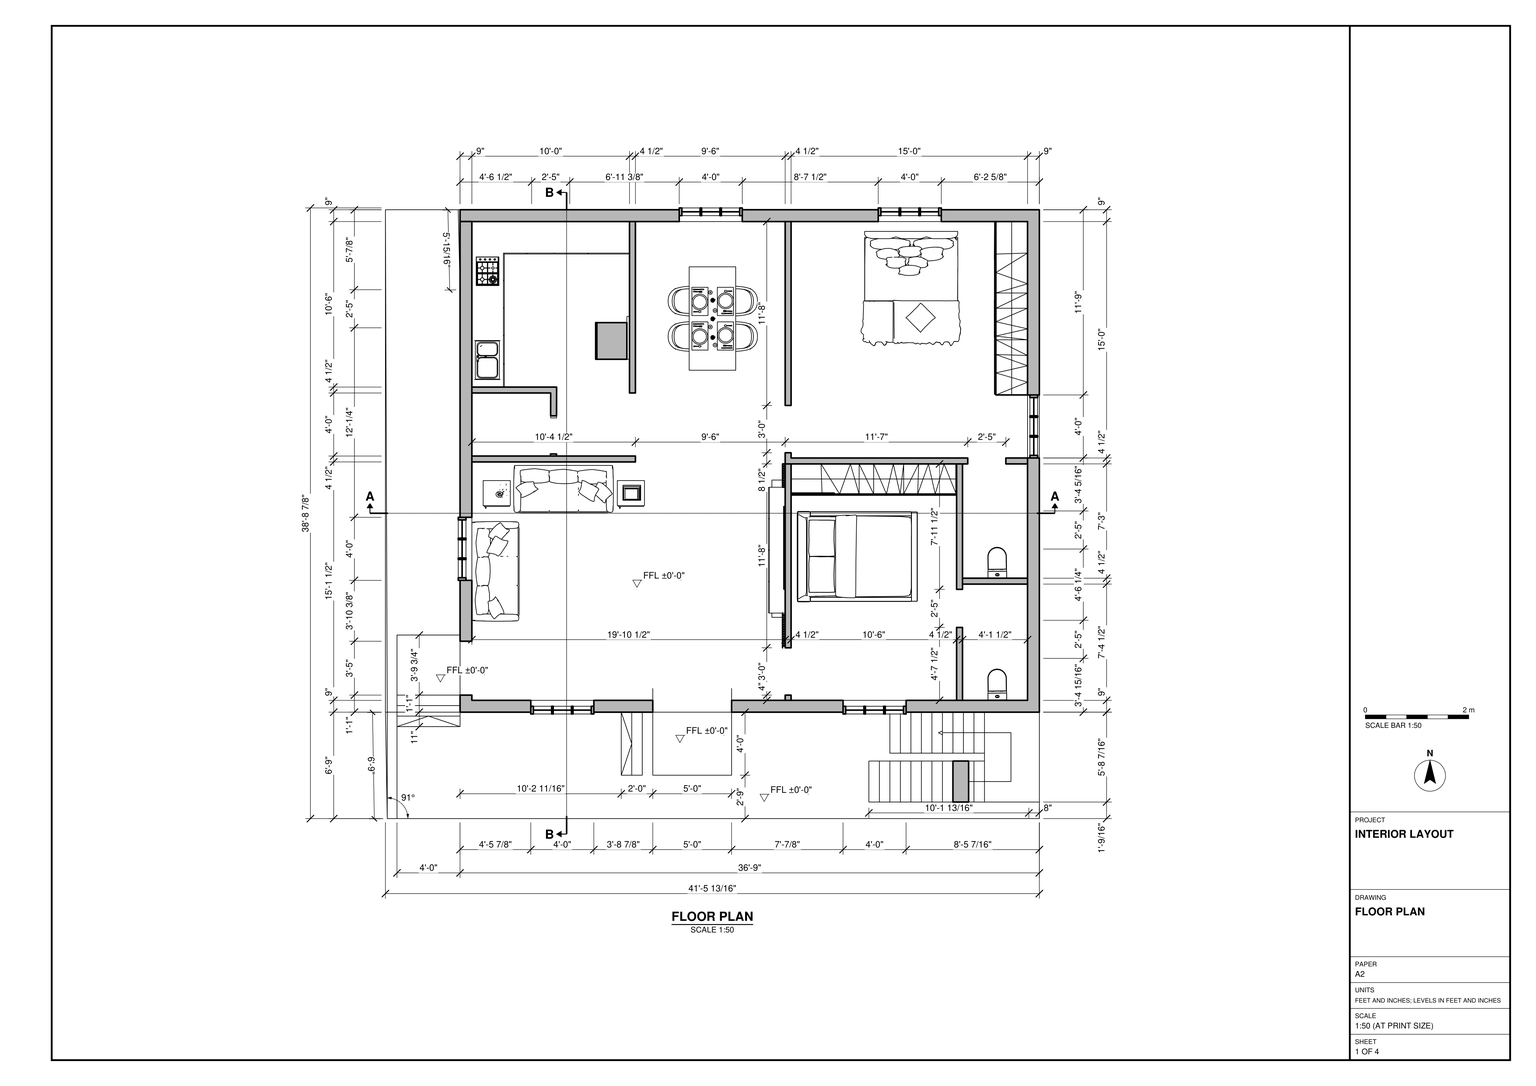
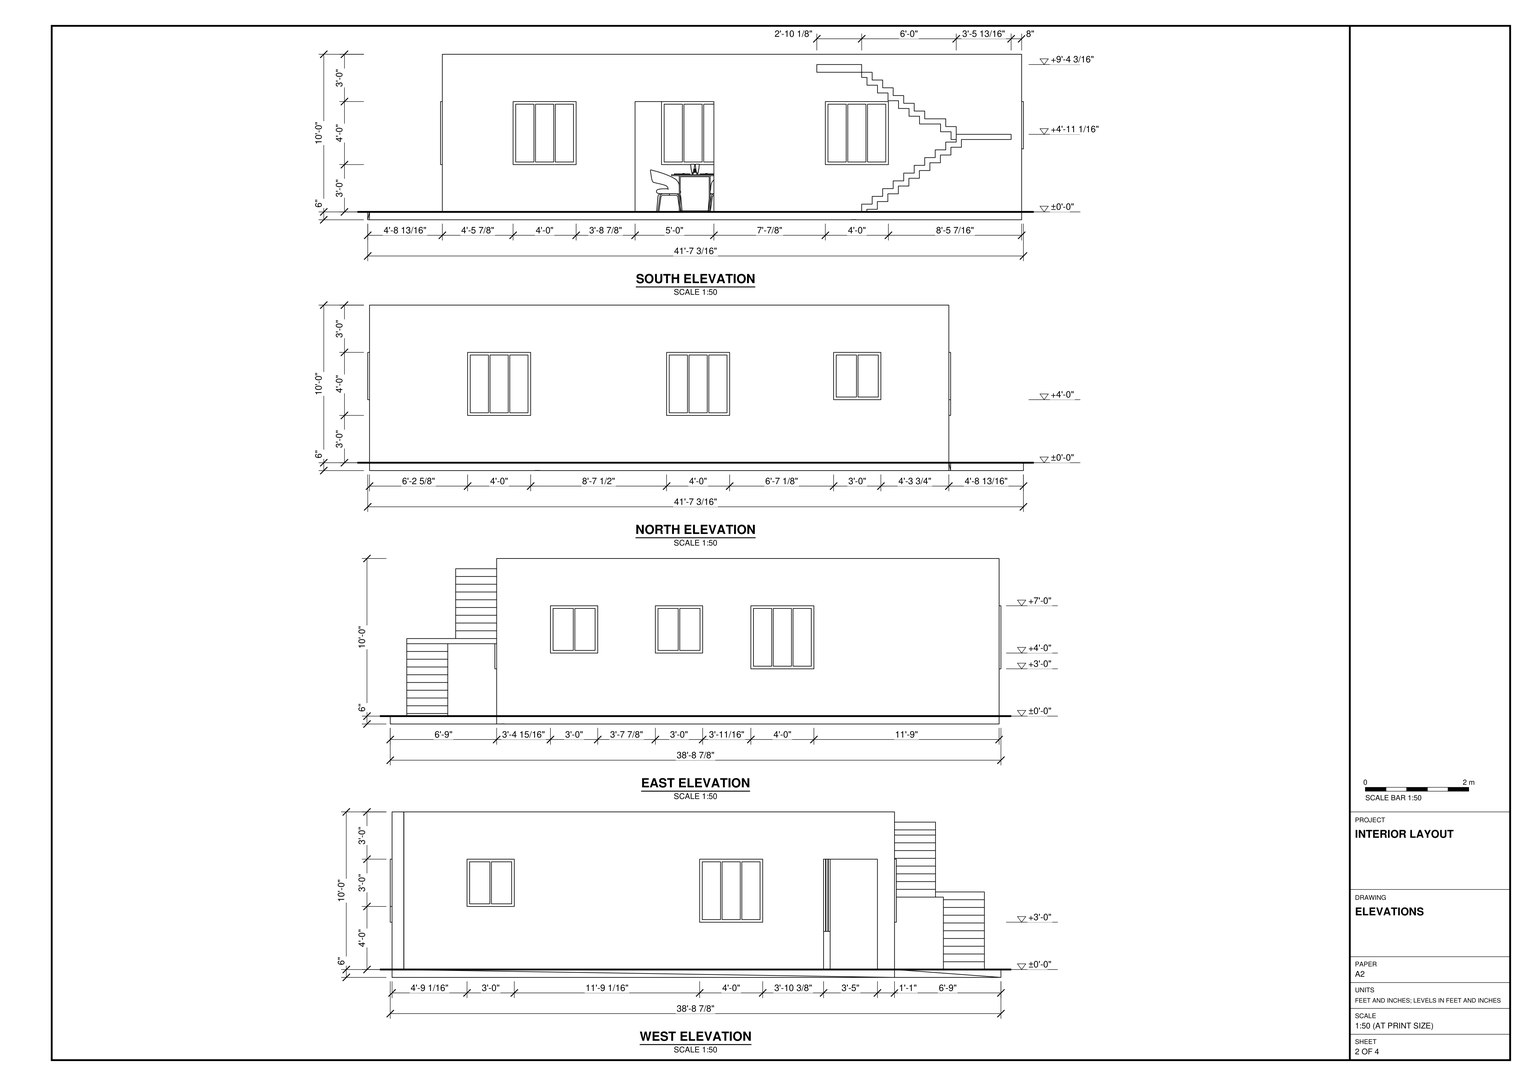
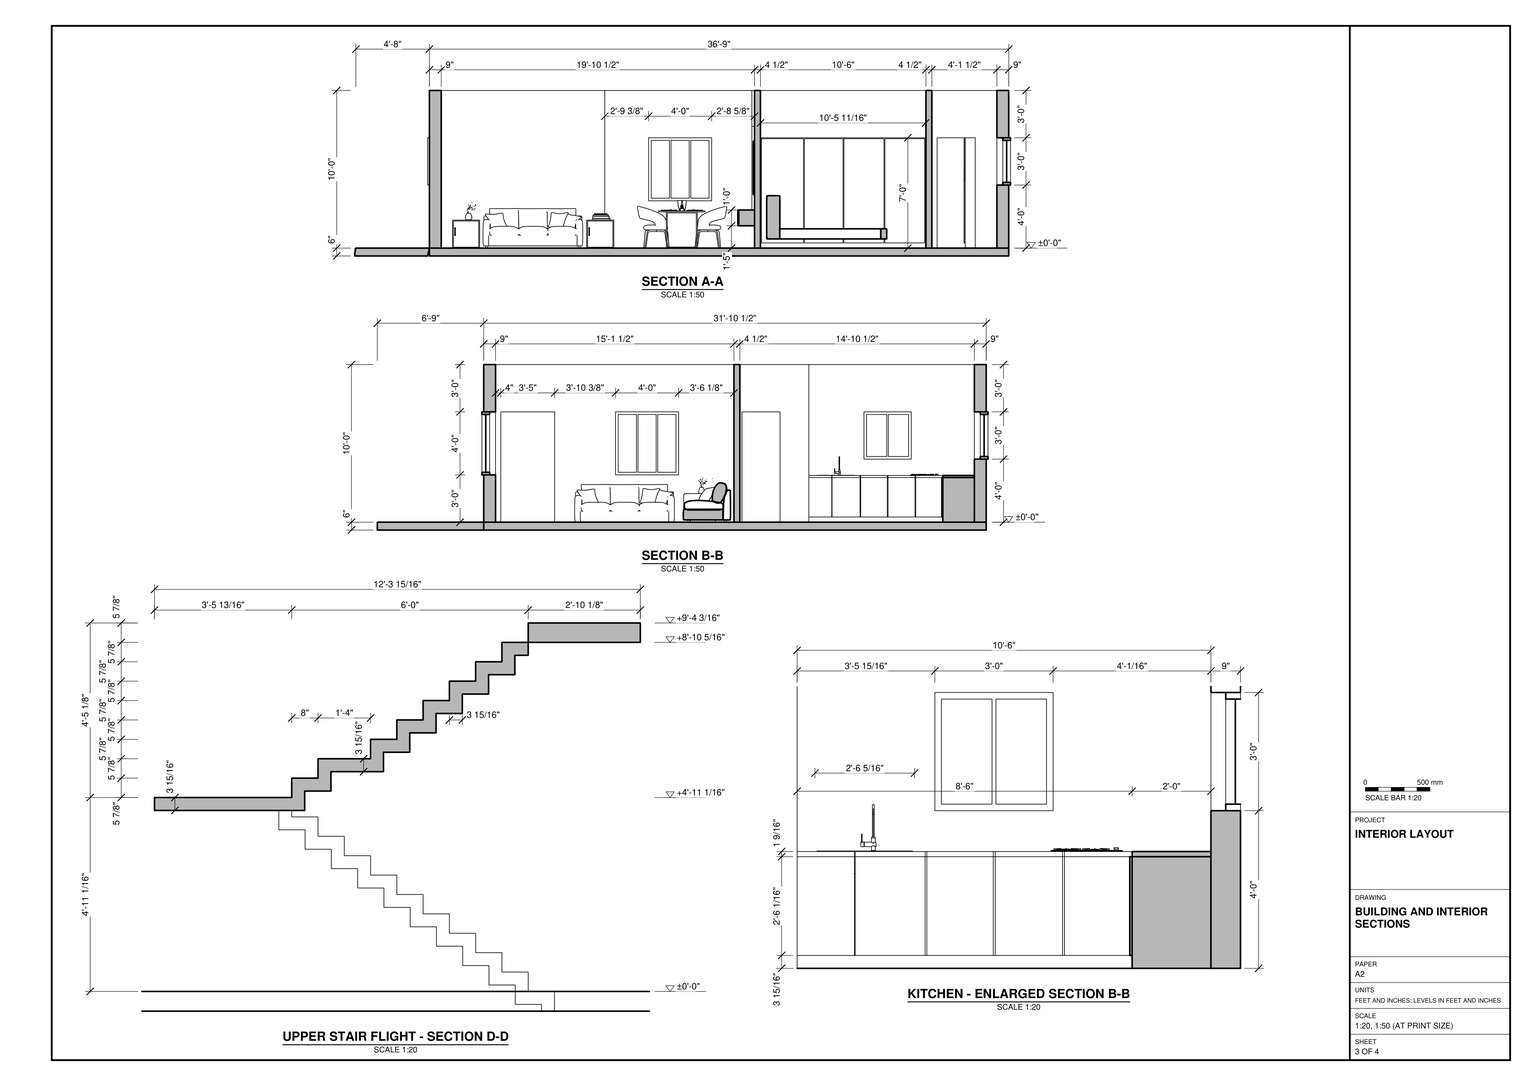
Build the single-storey residential layout in SketchUp from task_files/diagram_01.pdf. Work in feet and inches. Set the finished floor at ±0'-0". The overall model, including the projecting slab, is 41'-7 3/16" along x, 38'-8 7/8" along y and 10'-6" high.

Start with the 6" floor slab, including the portions extending beyond the south and west walls. Set out the 9" perimeter walls and the 4 1/2" partitions as drawn, with wall tops 10'-0" above the finished floor. Use the elevations to place the framed windows and exterior doorways. Build the exterior stair at the southeast corner with two flights that reverse direction at a shared landing.

Fit out the northwest kitchen with base cabinets, countertop, sink and cooktop. Place the dining table and chairs between the kitchen and the northeast bedroom, leaving the passage to the living area clear. Match the sofa arrangement in the southwest living area. Model both eastern bedrooms with their beds and fitted wardrobes, and include the two toilet compartments along the east wall.

Keep shell elements, the stair and each furniture or joinery piece in separate groups or components; use components for repeated parts. Decor and loose items, including lamps and appliances, may be any suitable library components. Save one SketchUp model as output_files/furnished_two_bedroom_layout_with_exterior_return_stair.skp.

# SketchUp Ruby script. Lengths in inches.
U = 1.inch
M = Sketchup.active_model
def pt(a) = Geom::Point3d.new(a.map { |v| v * U })
def face(e, loops, mat)
  f = e.add_face(loops[0].map { |a| pt(a) })
  loops[1..].each { |l| e.add_face(l.map { |a| pt(a) }).erase! }
  f.material = f.back_material = mat if mat
  f
end
# faces: each face lists its corners as indices into pts; further lists are holes
def faces(e, pts, list, mat = nil) = list.each { |f| face(e, (f[0].is_a?(Array) ? f : [f]).map { |l| l.map { |i| pts[i] } }, mat) }
# xy, xz, yz: faces in a plane at the given z, y or x. An outline is a flat list of corners, or four numbers for a rectangle; further outlines are holes
def ring(l) = l.size == 4 ? [[l[0], l[1]], [l[2], l[1]], [l[2], l[3]], [l[0], l[3]]] : l.each_slice(2).to_a
def flat(e, list, mat, &to3) = list.each { |f| face(e, (f[0].is_a?(Array) ? f : [f]).map { |l| ring(l).map { |u, v| to3.(u, v) } }, mat) }
def xy(e, z, list, mat = nil) = flat(e, list, mat) { |x, y| [x, y, z] }
def xz(e, y, list, mat = nil) = flat(e, list, mat) { |x, z| [x, y, z] }
def yz(e, x, list, mat = nil) = flat(e, list, mat) { |y, z| [x, y, z] }
def lines(e, pts, list) = list.each { |a, b| e.add_line(pt(pts[a]), pt(pts[b])) }
# prism: a flat outline (further loops are holes) pulled along v
def prism(e, loops, v, mat = nil)
  f = face(e, loops, mat); d = Geom::Vector3d.new(v.map { |x| x * U })
  f.pushpull(f.normal.samedirection?(d) ? d.length : -d.length)
end
def box(e, o, s, mat = nil) = prism(e, [[o, [o[0] + s[0], o[1], o[2]], [o[0] + s[0], o[1] + s[1], o[2]], [o[0], o[1] + s[1], o[2]]]], [0, 0, s[2]], mat)
def at(x, y, z, deg = 0) = Geom::Transformation.translation(pt([x, y, z])) * Geom::Transformation.rotation(ORIGIN, Z_AXIS, deg.degrees)
def axes(o, x, y, z) = Geom::Transformation.new([*x, 0, *y, 0, *z, 0, *pt(o).to_a, 1])
def part(name) = M.definitions.add(name)
# library, detail: a bought-in or finely detailed component or shape, given as its bounding box
def library(name, o, s) = part(name).tap { |d| box(d.entities, o, s) }
def detail(e, o, s) = box(e.add_group.entities, o, s)
def put(e, d, t, mat = nil) = e.add_instance(d, t).tap { |i| i.material = mat if mat }
def group(e, t, mat = nil) = e.add_group.tap { |g| g.transformation = t; g.material = mat if mat }.entities
root = M.entities
M.materials.add("2121 AP  X165 Dhaani-I").color = [217, 210, 92]
M.materials.add("2130 AP  X175 Sawan-I").color = [3, 168, 115]
M.materials.add("2186 AP  X202 Auspicious red-I").color = [192, 71, 86]
M.materials.add("Translucent_Glass_Gray1").color = [255, 255, 255]
M.materials["Translucent_Glass_Gray1"].alpha = 0.2
M.materials.add("Vicostone-BQ8740-Nero-Marquina-or-NERO-MARQUINAtm-CAN-or-US-").color = [21, 21, 22]
M.materials.add("[Chris_Shoe]").color = [23, 22, 22]
M.materials.add("[Color M05]").color = [114, 114, 114]
M.materials.add("[Color M08]").color = [30, 30, 30]
M.materials.add("[Color M09]").color = [0, 0, 0]
M.materials.add("[Tile Large Brown]").color = [193, 176, 158]
M.materials.add("[Translucent Glass Blue]").color = [100, 149, 237]
M.materials["[Translucent Glass Blue]"].alpha = 0.5
M.materials.add("[Wood Veneer 01]").color = [119, 69, 36]
c1 = part("new blockwindow")
p = [[-24,-4.5,0],[-24,4.5,0],[24,4.5,0],[24,-4.5,0],[24,-2,0],[-24,-2,0],
  [24,2,0],[-24,2,0]]
lines(c1.entities,p,[[0,1],[1,2],[2,3],[3,0],[4,5],[6,7]])
c2 = part("Bed - Queen")
p = [[22,23.6,0],[16.8,23.6,0],[22,38.8,0],[1.2,38.8,0],[1.2,25.6,0],[-1.2,38.8,0],
  [-1.2,25.6,0],[-22,38.8,0],[-22,25.6,0],[30,-40,0],[-30,-40,0],[-30,40,0],
  [14.8,23.2,0],[-30,23.2,0],[-30,25.6,0],[14.8,25.6,0],[30,40,0],[30,10.4,0],
  [14.8,10.4,0]]
lines(c2.entities,p,[[0,1],[2,0],[3,2],[4,3],[5,6],[7,5],[8,7],[9,10],[10,11],[12,13],[14,15],[11,16],
  [16,9],[17,15],[18,17],[15,18]])
c3 = library("Dining Set - 36 x 72 in.",[-45.5,-27.5,0],[91,55,0.01])
c4 = part("Sofa - Roundback 7 ft.")
p = [[12,-15.44,0],[12,10.4,0],[42,9,0],[42,-17,0],[36,-17,0],[36,5.53,0],
  [-12,-15.44,0],[-12,10.4,0],[-36,-17,0],[-42,-17,0],[-42,9,0],[-36,5.53,0],
  [-36,-15.44,0],[36,-15.44,0],[-36,3.62,0],[36,3.62,0],[28.96,7.49,0],[21.8125,9.02,0],
  [14.59,10.12,0],[7.31,10.78,0],[0,11,0],[-7.31,10.78,0],[-14.59,10.12,0],[-21.8125,9.02,0],
  [-28.96,7.49,0],[35.26,11.42,0],[28.37,13.42,0],[21.38,14.98,0],[14.3,16.1,0],[7.16,16.78,0],
  [0,17,0],[-7.16,16.78,0],[-14.3,16.1,0],[-21.38,14.98,0],[-28.37,13.42,0],[-35.26,11.42,0]]
lines(c4.entities,p,[[0,1],[2,3],[3,4],[4,5],[6,7],[8,9],[9,10],[8,11],[12,13],[14,15],[5,16],[16,17],
  [17,18],[18,19],[19,20],[20,21],[21,22],[22,23],[23,24],[24,11],[2,25],[25,26],[26,27],[27,28],
  [28,29],[29,30],[30,31],[31,32],[32,33],[33,34],[34,35],[35,10]])
c5 = library("Sink-double - 36 in top",[-18,-10.5,0],[36,21,0.01])
c6 = library("Range-Oven - 30 in top",[-15,-13,0],[30,26,0.01])
c7 = library("Dishwasher",[-12,-17.25,0],[24,34.5,0.01])
c8 = library("lamp",[-10.34,-9.52,0],[20.68,19.04,0.01])
c9 = library("Sofa 005",[-44.88,-17.99,0],[89.76,35.98,35.98])
c10 = library("1-POIGNEE CLC2",[-3.03,-0.375,0],[6.06,0.75,1.42])
c11 = library("2-VASEFLEURS CLC2",[-2.64,-4.18,0],[11.14,15.39,15.4375])
c12 = library("Stack of books",[0,0,0],[13.58,11.5,4.89])
c13 = part("Component\#1")
box(c13.entities,[0,0,0],[35.43,78.74,0.79],"Translucent_Glass_Gray1")
c14 = part("Rectangular frame")
prism(c14.entities,[[[29.53,5.91,0],[29.53,5.91,27.56],[5.91,5.91,27.56],[5.91,5.91,0]],[[28.74,5.91,0.79],[6.69,5.91,0.79],[6.69,5.91,26.77],[28.74,5.91,26.77]]],[0,3.9375,0],"[Color M08]")
c15 = library("chair 62",[0,0,0],[22.98,24.17,32.16])
c16 = library("Potted succulent",[-0.04,0,0],[3.63,3.68,4.41])
c17 = library("glass",[-1.4375,-1.4375,0],[2.875,2.875,7.95])
c18 = library("Bed 003",[-38.05,-87.1,0],[75.86,87.1,46.85])
c19 = library("Crowd Pleaser Bed",[-34.48,-45.67,0],[68.96,91.51,40.05])
c20 = library("Toilet",[-7.17,-23.62,0],[14.34,23.62,32.58])
c21 = part("Component")
g1 = group(c21.entities,at(263.61,28.98,0))
xy(g1,1.32,[[-23.76,-27.93,-22.86,0]])
xy(g1,30.41,[[-23.76,-24.34,-22.94,-3.73]])
xy(g1,32.16,[[-23.76,-27.93,-22.94,-24.34],[-23.76,-3.73,-22.94,0]])
xy(g1,32.68,[[-23.76,-27.93,-22.94,0]])
xy(g1,72.97,[[-23.76,-27.93,-22.86,0]])
xz(g1,-27.93,[[-23.76,1.32,-22.86,1.32,-22.86,72.97,-23.76,72.97,-23.76,32.68,-22.94,32.68,-22.94,32.16,-23.76,32.16]])
xz(g1,-24.34,[[-23.76,30.41,-22.94,32.16]])
xz(g1,-3.73,[[-23.76,30.41,-22.94,32.16]])
xz(g1,0,[[-23.76,1.32,-23.76,32.16,-22.94,32.16,-22.94,32.68,-23.76,32.68,-23.76,72.97,-22.86,72.97,-22.86,1.32]])
yz(g1,-23.76,[[-27.93,1.32,-27.93,32.16,-24.34,32.16,-24.34,30.41,-3.73,30.41,-3.73,32.16,0,32.16,0,1.32],[-27.93,32.68,0,72.97]])
yz(g1,-22.94,[[-24.34,30.41,-3.73,32.16],[-27.93,32.16,0,32.68]])
yz(g1,-22.86,[[-27.93,1.32,0,72.97]])
g2 = group(g1,at(-22.86,-1.74,75.13))
xy(g2,-75.13,[[0,-26.1875,22.86,1.72]])
xy(g2,-2.16,[[0,-26.1875,22.86,1.72]])
xz(g2,-26.1875,[[0,-75.13,22.86,-2.16]])
xz(g2,1.72,[[0,-75.13,22.86,-2.16]])
yz(g2,0,[[-26.1875,-75.13,1.72,-73.81],[1.72,-75.13,1.74,-73.81],[-26.1875,-73.81,1.72,-2.16]])
yz(g2,22.86,[[-26.1875,-75.13,1.72,-2.16]])
c22 = library("4-TABLE DE CUISSON CLC2",[-10.93,-8.66,0.2],[21.86,17.32,1.1])
c23 = library("2-EVIER M80 CLC2\#1",[-15.14,-9.87,-6.7],[30.32,19.69,21.06])
c24 = part("Group18\#1")
xy(c24.entities,0,[[121.34,276.07,116.84,276.08,116.84,277.59,121.34,277.58],[121.43,306.58,116.93,306.59,116.99,324,57,324,57,328.5,121.5,328.5]])
xy(c24.entities,84,[[121.34,277.58,116.84,277.59,116.93,306.59,121.43,306.58]])
xy(c24.entities,120,[[121.34,276.07,121.5,328.5,57,328.5,57,324,116.99,324,116.84,276.08]])
xz(c24.entities,324,[[57,0,116.99,120]])
xz(c24.entities,328.5,[[57,0,121.5,120]])
yz(c24.entities,57,[[324,0,328.5,120]])
# 1 loose lines left out
p = [[116.99,324,0],[116.93,306.59,0],[116.93,306.59,84],[116.84,277.59,84],[116.84,277.59,0],[116.84,276.08,0],
  [116.84,276.08,120],[116.99,324,120],[121.34,276.07,0],[121.34,276.07,120],[121.34,277.58,0],[121.34,277.58,84],
  [121.43,306.58,84],[121.43,306.58,0],[121.5,328.5,0],[121.5,328.5,120]]
faces(c24.entities,p,[[0,1,2,3,4,5,6,7],[8,9,6,5],[8,10,11,12,13,14,15,9],[4,3,11,10],[2,1,13,12]])
c25 = part("Group19\#1")
box(c25.entities,[57,271.5,0],[124.5,4.5,120])
c26 = part("Group21\#1")
box(c26.entities,[177,324,0],[4.5,130.5,120])
c27 = part("Group22\#1")
xy(c27.entities,0,[[295.5,270,295.5,278.5,300,278.5,300,274.5,434.5,274.5,434.5,270],[463.5,270,480,274.5],[295.5,314.5,300,454.5]])
xy(c27.entities,84,[[434.5,270,463.5,274.5],[295.5,278.5,300,314.5]])
xy(c27.entities,120,[[295.5,270,480,270,480,274.5,300,274.5,300,454.5,295.5,454.5]])
xz(c27.entities,270,[[295.5,0,434.5,0,434.5,84,463.5,84,463.5,0,480,0,480,120,295.5,120]])
xz(c27.entities,274.5,[[300,0,300,120,480,120,480,0,463.5,0,463.5,84,434.5,84,434.5,0]])
xz(c27.entities,278.5,[[295.5,0,300,84]])
xz(c27.entities,314.5,[[295.5,0,300,84]])
xz(c27.entities,454.5,[[295.5,0,300,120]])
yz(c27.entities,295.5,[[270,0,270,120,454.5,120,454.5,0,314.5,0,314.5,84,278.5,84,278.5,0]])
yz(c27.entities,300,[[274.5,0,278.5,0,278.5,84,314.5,84,314.5,0,454.5,0,454.5,120,274.5,120]])
yz(c27.entities,434.5,[[270,0,274.5,84]])
yz(c27.entities,463.5,[[270,0,274.5,84]])
yz(c27.entities,480,[[270,0,274.5,120]])
c28 = part("Group24\#1")
prism(c28.entities,[[[430.5,90,0],[430.5,145.5,0],[430.5,145.5,84],[430.5,174.5,84],[430.5,174.5,0],[430.5,270,0],[430.5,270,120],[430.5,90,120]]],[-4.5,0,0])
c29 = part("Group26\#1")
box(c29.entities,[430.5,178.5,0],[49.5,4.5,120])
c30 = library("Group\#2",[0,0,0],[100.17,68.42,0.01])
c31 = library("Group\#3",[0,0,0],[121.79,68.42,0.01])
c32 = library("Group\#6",[0,0,0],[121.79,68.42,118.11])
c33 = part("Group55\#3")
xy(c33.entities,0,[[-22,-22,-8.125,22],[-6.9375,-22,6.9375,22],[8.125,-22,22,22]])
c34 = part("Group54\#1")
prism(c34.entities,[[[-24,24,0],[24,24,0],[24,-24,0],[-24,-24,0]],[[-22,22,0],[-22,-22,0],[-8.125,-22,0],[-8.125,22,0]],[[6.9375,22,0],[-6.9375,22,0],[-6.9375,-22,0],[6.9375,-22,0]],[[22,-22,0],[22,22,0],[8.125,22,0],[8.125,-22,0]]],[0,0,5.875],"[Chris_Shoe]")
put(c34.entities,c33,at(0,0,2.9375))
c35 = part("Group57\#2")
xy(c35.entities,0,[[-22,-22,-8.125,22],[-6.9375,-22,6.9375,22],[8.125,-22,22,22]])
c36 = part("Group56\#1")
prism(c36.entities,[[[24,-24,0],[-24,-24,0],[-24,24,0],[24,24,0]],[[-22,22,0],[-22,-22,0],[-8.125,-22,0],[-8.125,22,0]],[[8.125,-22,0],[22,-22,0],[22,22,0],[8.125,22,0]],[[-6.9375,-22,0],[6.9375,-22,0],[6.9375,22,0],[-6.9375,22,0]]],[0,0,5.875],"[Chris_Shoe]")
put(c36.entities,c35,at(0,0,2.9375))
c37 = part("Group54\#2")
prism(c37.entities,[[[-24,24,0],[24,24,0],[24,-24,0],[-24,-24,0]],[[-22,22,0],[-22,-22,0],[-8.125,-22,0],[-8.125,22,0]],[[6.9375,22,0],[-6.9375,22,0],[-6.9375,-22,0],[6.9375,-22,0]],[[22,-22,0],[22,22,0],[8.125,22,0],[8.125,-22,0]]],[0,0,5.875],"[Chris_Shoe]")
put(c37.entities,c33,at(0,0,2.9375))
c38 = part("Group63\#2")
xy(c38.entities,0,[[-22,-22,-8.125,22],[-6.9375,-22,6.9375,22],[8.125,-22,22,22]])
c39 = part("Group62\#2")
prism(c39.entities,[[[-24,-24,0],[-24,24,0],[24,24,0],[24,-24,0]],[[6.9375,22,0],[-6.9375,22,0],[-6.9375,-22,0],[6.9375,-22,0]],[[8.125,22,0],[8.125,-22,0],[22,-22,0],[22,22,0]],[[-8.125,-22,0],[-8.125,22,0],[-22,22,0],[-22,-22,0]]],[0,0,5.875],"[Chris_Shoe]")
put(c39.entities,c38,at(0,0,2.9375))
c40 = part("Group65\#3")
xy(c40.entities,0,[[-22,-22,-8.125,22],[-6.9375,-22,6.9375,22],[8.125,-22,22,22]])
c41 = part("Group64\#1")
prism(c41.entities,[[[-24,-24,0],[-24,24,0],[24,24,0],[24,-24,0]],[[-6.9375,-22,0],[6.9375,-22,0],[6.9375,22,0],[-6.9375,22,0]],[[8.125,-22,0],[22,-22,0],[22,22,0],[8.125,22,0]],[[-22,-22,0],[-8.125,-22,0],[-8.125,22,0],[-22,22,0]]],[0,0,5.875],"[Chris_Shoe]")
put(c41.entities,c40,at(0,0,2.9375))
c42 = part("Group67\#2")
xy(c42.entities,0,[[-16,-16,-0.59,16],[0.59,-16,16,16]])
c43 = part("Group66\#1")
prism(c43.entities,[[[-18,18,0],[18,18,0],[18,-18,0],[-18,-18,0]],[[16,-16,0],[16,16,0],[0.59,16,0],[0.59,-16,0]],[[-0.59,16,0],[-16,16,0],[-16,-16,0],[-0.59,-16,0]]],[0,0,5.875],"[Chris_Shoe]")
put(c43.entities,c42,at(0,0,2.9375))
c44 = part("Group69\#3")
xy(c44.entities,0,[[-16,-16,-0.59,16],[0.59,-16,16,16]])
c45 = part("Group68\#1")
prism(c45.entities,[[[-18,18,0],[18,18,0],[18,-18,0],[-18,-18,0]],[[-16,-16,0],[-0.59,-16,0],[-0.59,16,0],[-16,16,0]],[[16,-16,0],[16,16,0],[0.59,16,0],[0.59,-16,0]]],[0,0,5.875],"[Chris_Shoe]")
put(c45.entities,c44,at(0,0,2.9375))
c46 = part("Group67\#3")
xy(c46.entities,0,[[-16,-16,-0.59,16],[0.59,-16,16,16]])
c47 = part("Group66\#2")
prism(c47.entities,[[[-18,18,0],[18,18,0],[18,-18,0],[-18,-18,0]],[[-16,-16,0],[-0.59,-16,0],[-0.59,16,0],[-16,16,0]],[[16,16,0],[0.59,16,0],[0.59,-16,0],[16,-16,0]]],[0,0,5.875],"[Chris_Shoe]")
put(c47.entities,c46,at(0,0,2.9375))
c48 = part("Group69\#4")
xy(c48.entities,0,[[-16,-16,-0.59,16],[0.59,-16,16,16]])
c49 = part("Group68\#2")
prism(c49.entities,[[[-18,18,0],[18,18,0],[18,-18,0],[-18,-18,0]],[[0.59,-16,0],[16,-16,0],[16,16,0],[0.59,16,0]],[[-0.59,-16,0],[-0.59,16,0],[-16,16,0],[-16,-16,0]]],[0,0,5.875],"[Chris_Shoe]")
put(c49.entities,c48,at(0,0,2.9375))
c50 = part("Group71\#2")
xy(c50.entities,0,[[-22,-22,-8.125,22],[-6.9375,-22,6.9375,22],[8.125,-22,22,22]])
c51 = part("Group70\#1")
xy(c51.entities,0,[[[-24,-24,24,24],[-22,-22,-8.125,22],[-6.9375,-22,6.9375,22],[8.125,-22,22,22]]])
xy(c51.entities,5.875,[[[-24,-24,24,24],[-22,-22,-8.125,22],[-6.9375,-22,6.9375,22],[8.125,-22,22,22]]],"[Chris_Shoe]")
xz(c51.entities,-24,[[-24,0,24,5.875]])
xz(c51.entities,-22,[[-22,0,-8.125,5.875],[-6.9375,0,6.9375,5.875],[8.125,0,22,5.875]])
xz(c51.entities,22,[[-22,0,-8.125,5.875],[-6.9375,0,6.9375,5.875],[8.125,0,22,5.875]])
xz(c51.entities,24,[[-24,0,24,5.875]])
yz(c51.entities,-24,[[-24,0,24,5.875]])
yz(c51.entities,-22,[[-22,0,22,5.875]])
yz(c51.entities,-8.125,[[-22,0,22,5.875]])
yz(c51.entities,-6.9375,[[-22,0,22,5.875]])
yz(c51.entities,6.9375,[[-22,0,22,5.875]])
yz(c51.entities,8.125,[[-22,0,22,5.875]])
yz(c51.entities,22,[[-22,0,22,5.875]])
yz(c51.entities,24,[[-24,0,24,5.875]])
put(c51.entities,c50,at(0,0,2.9375))
c52 = part("Group")
xy(c52.entities,0,[[0,0,20.67,19.04]])
xy(c52.entities,0.71,[[0.71,-0.71,19.96,0]])
xy(c52.entities,20.61,[[0.71,-0.71,19.96,0]])
xy(c52.entities,21.32,[[0,0,20.67,19.04]])
xz(c52.entities,-0.71,[[0.71,0.71,19.96,20.61]])
xz(c52.entities,0,[[[0,0,20.67,21.32],[0.71,0.71,19.96,20.61]]])
xz(c52.entities,19.04,[[0,0,20.67,21.32]])
yz(c52.entities,0,[[0,0,19.04,21.32]])
yz(c52.entities,0.71,[[-0.71,0.71,0,20.61]])
yz(c52.entities,19.96,[[-0.71,0.71,0,20.61]])
yz(c52.entities,20.67,[[0,0,19.04,21.32]])
c53 = part("Group\#13")
box(c53.entities,[0,0,0],[21.5,12.25,0.2])
c54 = library("Group\#12",[0,0,0],[18.06,12.04,0.75])
c55 = library("Group150\#1",[-70,-45.5,0],[140,91,2])
c56 = part("Group23\#1")
xy(c56.entities,0,[[295.5,90,300,94],[295.5,130,300,270]])
xy(c56.entities,84,[[295.5,94,300,130]])
xy(c56.entities,120,[[295.5,90,300,270]])
xz(c56.entities,90,[[295.5,0,300,120]])
xz(c56.entities,94,[[295.5,0,300,84]])
xz(c56.entities,130,[[295.5,0,300,84]])
xz(c56.entities,270,[[295.5,0,300,120]])
yz(c56.entities,295.5,[[90,0,90,120,130,120,130,84,94,84,94,0],[130,0,270,120]])
yz(c56.entities,300,[[90,0,94,0,94,84,130,84,130,0,270,0,270,120,90,120]])
c57 = part("Group16\#1")
xy(c57.entities,0,[[254.71,81,489,81,489,463.5,48,463.5,48,454.5,480,454.5,480,90,254.71,90],[48,81,194.71,81,194.71,90,57,90,57,94,48,94],[48,135,57,454.59]])
xy(c57.entities,36,[[101.86,81,149.86,90],[339.5625,81,387.5625,90],[48,181.35,57,229.35],[480,274.5,489,322.5],[214.85,454.5,262.85,463.5],
  [366.35,454.5,414.35,463.5]])
xy(c57.entities,48,[[480,121.94,489,157.94],[480,201.8125,489,237.8125],[48,370.44,57,406.44],[99.72,454.5,135.72,463.5]])
xy(c57.entities,84,[[101.86,81,149.86,90],[194.71,81,254.71,90],[339.5625,81,387.5625,90],[48,94,57,135],[480,121.94,489,157.94],
  [48,181.35,57,229.35],[480,201.8125,489,237.8125],[480,274.5,489,322.5],[48,370.44,57,406.44],[99.72,454.5,135.72,463.5],
  [214.85,454.5,262.85,463.5],[366.35,454.5,414.35,463.5]])
xy(c57.entities,120,[[48,81,48,454.59,57,454.59,57,90,480,90,480,454.5,48,454.5,48,463.5,489,463.5,489,81]])
xz(c57.entities,81,[[[48,0,48,120,489,120,489,0,254.71,0,254.71,84,194.71,84,194.71,0],[101.86,36,149.86,84],[339.5625,36,387.5625,84]]])
xz(c57.entities,90,[[[57,0,194.71,0,194.71,84,254.71,84,254.71,0,480,0,480,120,57,120],[101.86,36,149.86,84],[339.5625,36,387.5625,84]]])
xz(c57.entities,94,[[48,0,57,84]])
xz(c57.entities,121.94,[[480,48,489,84]])
xz(c57.entities,135,[[48,0,57,84]])
xz(c57.entities,157.94,[[480,48,489,84]])
xz(c57.entities,181.35,[[48,36,57,84]])
xz(c57.entities,201.8125,[[480,48,489,84]])
xz(c57.entities,229.35,[[48,36,57,84]])
xz(c57.entities,237.8125,[[480,48,489,84]])
xz(c57.entities,274.5,[[480,36,489,84]])
xz(c57.entities,322.5,[[480,36,489,84]])
xz(c57.entities,370.44,[[48,48,57,84]])
xz(c57.entities,406.44,[[48,48,57,84]])
xz(c57.entities,454.5,[[[48,0,480,120],[214.85,36,262.85,84],[366.35,36,414.35,84],[99.72,48,135.72,84]]])
xz(c57.entities,454.59,[[48,0,57,120]])
xz(c57.entities,463.5,[[[48,0,489,120],[214.85,36,262.85,84],[366.35,36,414.35,84],[99.72,48,135.72,84]]])
yz(c57.entities,48,[[[81,0,94,0,94,84,135,84,135,0,454.59,0,454.59,120,81,120],[181.35,36,229.35,84],[370.44,48,406.44,84]],[454.5,0,463.5,120]])
yz(c57.entities,57,[[[90,0,94,0,94,84,135,84,135,0,454.59,0,454.59,120,90,120],[181.35,36,229.35,84],[370.44,48,406.44,84]]])
yz(c57.entities,99.72,[[454.5,48,463.5,84]])
yz(c57.entities,101.86,[[81,36,90,84]])
yz(c57.entities,135.72,[[454.5,48,463.5,84]])
yz(c57.entities,149.86,[[81,36,90,84]])
yz(c57.entities,194.71,[[81,0,90,84]])
yz(c57.entities,214.85,[[454.5,36,463.5,84]])
yz(c57.entities,254.71,[[81,0,90,84]])
yz(c57.entities,262.85,[[454.5,36,463.5,84]])
yz(c57.entities,339.5625,[[81,36,90,84]])
yz(c57.entities,366.35,[[454.5,36,463.5,84]])
yz(c57.entities,387.5625,[[81,36,90,84]])
yz(c57.entities,414.35,[[454.5,36,463.5,84]])
yz(c57.entities,480,[[[90,0,454.5,120],[274.5,36,322.5,84],[201.8125,48,237.8125,84],[121.94,48,157.94,84]]])
yz(c57.entities,489,[[[81,0,463.5,120],[274.5,36,322.5,84],[201.8125,48,237.8125,84],[121.94,48,157.94,84]]])
# 5 loose lines left out
box(root,[341.875,49.79,106.3],[34.14,31.21,5.9])
xy(root,-6,[[1.38,0,0,81,497.81,81,497.81,0],[0,81,55.42,463.5]])
xy(root,0,[[1.38,0,8.81,81],[8.81,0,497.81,0,497.81,12.58,376.02,12.58,376.02,43.79,456.02,43.79,456.02,49.79,384.02,49.79,384.02,81,263.52,81,263.52,33,203.52,33,203.52,81,195.52,81,195.52,33,179.52,33,179.52,81,56.81,81,56.81,70,8.81,70],[376.02,12.58,384.02,28.1875],[384.02,12.58,392.02,28.1875],[392.02,12.58,400.02,28.1875],
  [400.02,12.58,408.02,28.1875],[408.02,12.58,416.02,28.1875],[416.02,12.58,424.02,28.1875],[424.02,12.58,432.02,28.1875],[432.02,12.58,440.02,28.1875],
  [440.02,12.58,448.02,28.1875],[448.02,12.58,456.02,28.1875],[456.02,12.58,497.81,12.58,497.81,81,456.02,81,456.02,65.4,476.1875,65.4,476.1875,28.1875,456.02,28.1875],[376.02,28.1875,384.02,43.79],[384.02,28.1875,392.02,43.79],
  [392.02,28.1875,400.02,43.79],[400.02,28.1875,408.02,43.79],[408.02,28.1875,416.02,43.79],[416.02,28.1875,424.02,43.79],[424.02,28.1875,432.02,43.79],
  [432.02,28.1875,440.02,43.79],[440.02,28.1875,448.02,43.79],[448.02,28.1875,456.02,43.79],[456.02,28.1875,476.1875,65.4],[179.52,33,187.52,33,187.52,57],
  [179.52,33,187.52,57,179.52,81],[187.52,33,195.52,81],[203.52,33,263.52,81],[384.02,49.79,392.02,81],[392.02,49.79,400.02,81],
  [400.02,49.79,408.02,81],[408.02,49.79,416.02,81],[416.02,49.79,424.02,49.79,424.02,63.74,420.98,65.4,424.02,66.6875,424.02,81,416.02,81],[424.02,49.79,432.02,65.4],[432.02,49.79,440.02,49.79,440.02,65.4,448.02,65.4,448.02,81,440.02,81,440.02,65.4,432.02,65.4],
  [440.02,49.79,448.02,65.4],[448.02,49.79,456.02,65.4],[187.52,57,187.52,81,179.52,81],[424.02,63.74,424.02,65.4,432.02,65.4,432.02,81,424.02,81,424.02,66.6875,420.98,65.4],[432.02,65.4,440.02,81],
  [448.02,65.4,456.02,81],[8.81,70,32.81,78,8.81,78],[8.81,70,56.81,70,32.81,78],[56.81,70,56.81,78,32.81,78],[8.81,78,56.81,81],
  [1.38,81,8.81,81,8.81,139.73,56.81,139.73,56.81,402.61,55.42,463.5,0,463.5],[8.81,81,56.81,86],[263.52,81,497.81,81,497.81,121.94,488.81,121.94,488.81,90,439.31,90,439.31,145.5,434.81,145.5,434.81,90,308.81,90,308.81,94,304.31,94,304.31,90,263.52,90],[8.81,86,56.81,94],[8.81,94,56.81,139.73],
  [56.81,135,65.81,135,65.81,271.5,190.31,271.5,190.31,276,65.81,276,65.81,324,125.81,324,125.81,305,130.31,305,130.31,328.5,64.42,328.5,64.42,373.61,56.81,373.61],[488.81,234.2,497.81,234.2,497.81,463.5,140.31,463.5,140.31,454.5,185.81,454.5,185.81,324,190.31,324,190.31,454.5,304.31,454.5,304.31,314.5,308.81,314.5,308.81,454.5,488.81,454.5,488.81,274.5,472.31,274.5,472.31,270,488.81,270],[464.7,322.5,476.75,322.5,476.75,327.375],[464.7,322.5,476.75,327.375,476.75,335.76,464.7,339.27],[476.75,322.5,488.81,322.5,488.81,332.25,476.75,327.375],
  [488.81,332.25,488.81,344.73,476.75,342,476.75,335.76],[464.7,339.27,476.75,342,476.75,349.02,464.7,353.31],[476.75,342,488.81,344.73,476.75,349.02],[488.81,344.73,488.81,352.53,476.75,352.92,476.75,349.02],[476.75,349.02,476.75,352.92,464.7,353.31],
  [488.81,352.53,476.75,358.51,476.75,352.92],[488.81,352.53,488.81,364.5,476.75,364.5,476.75,358.51],[476.75,352.92,476.75,358.51,464.7,364.5,464.7,353.31],[476.75,358.51,476.75,364.5,464.7,364.5],[464.7,364.5,476.75,364.5,476.75,365.92,464.7,367.35],
  [476.75,364.5,488.81,364.5,476.75,365.92],[488.81,364.5,488.81,372.81,476.75,370.08,476.75,365.92],[476.75,365.92,476.75,370.08,464.7,367.35],[464.7,367.35,476.75,370.08,476.75,375.54,464.7,378.27],[476.75,370.08,488.81,372.81,476.75,375.54],
  [488.81,372.81,488.81,388.5,476.75,383.38,476.75,375.54],[63.31,373.61,64.42,402.61],[476.75,375.54,476.75,383.38,464.7,378.27],[464.7,378.27,476.75,383.38,476.75,388.5,464.7,388.5],[476.75,383.38,488.81,388.5,476.75,388.5],
  [464.7,388.5,476.75,388.5,476.75,394.31],[464.7,388.5,476.75,394.31,476.75,400.11,464.7,400.11],[476.75,388.5,488.81,388.5,488.81,400.11,476.75,394.31],[476.75,394.31,488.81,400.11,476.75,400.11],[464.7,400.11,476.75,400.11,476.75,403.62],
  [464.7,400.11,476.75,403.62,476.75,411.42,464.7,415.71],[476.75,400.11,488.81,400.11,488.81,407.13,476.75,403.62],[56.81,402.61,64.42,402.61,64.42,454.5,111.31,454.5,111.31,463.5,55.42,463.5],[476.75,403.62,488.81,407.13,476.75,411.42],[488.81,407.13,488.81,430.53,476.75,423.12,476.75,411.42],
  [476.75,411.42,476.75,423.12,464.7,415.71],[464.7,415.71,476.75,423.12,476.75,430.14,464.7,429.75],[464.7,429.75,476.75,430.14,476.75,454.5,464.7,454.5],[476.75,430.14,488.81,430.53,488.81,454.5,476.75,454.5],[111.31,454.5,140.31,457]])
xy(root,3.9375,[[309.51,246.33,341.58,247.75],[342.29,246.33,371.66,247.04],[372.37,246.33,402.85,247.04],[403.56,246.33,433.81,247.04],[89.81,328.5,90.51,367.47],
  [89.81,367.99,90.51,388.22],[89.81,388.8125,90.51,409.3],[89.81,409.9,90.51,430.5],[90.51,429.79,107.25,430.5],[107.71,429.79,128.18,430.5],
  [128.91,429.79,153.77,430.5],[154.25,429.79,185.81,430.5]])
xy(root,3.96,[[463.8,366.09,464.51,395.09]])
xy(root,4.04,[[464.51,425.5,463.8,425.51,463.99,453.8,464.7,453.79]])
xy(root,4.14,[[89.81,345.9375,90.51,346.17]])
xy(root,17,[[292.31,156.43,304.31,252.24],[291.6,156.59,292.31,180.27],[291.6,180.5,292.31,204.22],[291.6,204.45,292.31,228.17],[291.6,228.4,292.31,252.16]])
xy(root,29,[[291.6,156.59,292.31,180.27]])
xy(root,29,[[292.31,156.43,304.31,252.24],[291.6,180.5,292.31,204.22],[291.6,204.45,292.31,228.17],[291.6,228.4,292.31,252.16]],"[Wood Veneer 01]")
xy(root,34,[[[64.42,328.5,64.42,454.5,185.81,454.5,185.81,430.5,89.81,430.5,89.81,328.5],[73.08,335.97,82.47,335.97,82.74,336.01,82.81,336.02,83.07,336.09,83.13,336.11,83.39,336.21,83.44,336.24,83.68,336.36,83.74,336.4,83.96,336.55,84.01,336.6,84.21,336.78,84.39,336.98,84.43,337.03,84.59,337.26,84.62,337.3125,84.75,337.56,84.78,337.61,84.87,337.87,84.89,337.93,84.95,338.2,84.97,338.26,85,338.53,85,348.07,84.96,348.36,84.95,348.43,84.87,348.72,84.85,348.79,84.74,349.06,84.71,349.125,84.57,349.38,84.53,349.45,84.35,349.68,84.3125,349.74,84.1,349.95,84.05,350,84,350.04,83.77,350.23,83.71,350.26,83.45,350.41,83.39,350.44,83.12,350.5625,83.05,350.58,82.77,350.66,82.7,350.67,82.41,350.72,73.17,350.72,73.09,350.71,72.79,350.69,72.72,350.68,72.43,350.62,72.36,350.6,72.08,350.5,72.02,350.47,71.75,350.34,71.69,350.3,71.44,350.14,71.39,350.09,71.17,349.89,70.97,349.67,70.92,349.62,70.76,349.37,70.72,349.31,70.59,349.04,70.55,348.98,70.46,348.7,70.43,348.63,70.375,348.34,70.36,348.27,70.34,347.96,70.33,347.89,70.33,338.5,70.37,338.23,70.38,338.16,70.45,337.9,70.47,337.83,70.57,337.58,70.6,337.52,70.73,337.28,70.77,337.22,70.93,337,70.97,336.94,71.16,336.74,71.21,336.7,71.26,336.65,71.47,336.48,71.53,336.44,71.76,336.3,71.82,336.27,72.07,336.15,72.13,336.13,72.4,336.05,72.46,336.04,72.73,335.99,72.8,335.98],[72.78,352.62,82.36,352.62,82.65,352.65,82.72,352.67,83.01,352.73,83.07,352.75,83.35,352.86,83.41,352.89,83.67,353.03,83.73,353.0625,83.96,353.24,84.01,353.28,84.23,353.48,84.41,353.71,84.46,353.76,84.61,354.01,84.64,354.0625,84.76,354.33,84.79,354.39,84.87,354.67,84.89,354.73,84.9375,355.02,84.95,355.08,84.95,359.5625,84.93,359.82,84.93,359.875,84.875,360.125,84.86,360.18,84.78,360.42,84.76,360.47,84.65,360.7,84.62,360.74,84.48,360.96,84.45,361,84.28,361.19,84.2,361.27,84.01,361.44,83.96,361.47,83.75,361.62,83.7,361.64,83.47,361.76,83.42,361.78,83.18,361.87,83.12,361.88,82.875,361.94,82.8125,361.95,82.56,361.98,72.78,361.98,72.71,361.97,72.46,361.95,72.4,361.93,72.15,361.875,72.1,361.86,71.86,361.77,71.58,361.63,71.53,361.6,71.32,361.45,71.27,361.42,71.08,361.25,70.92,361.0625,70.875,361.02,70.73,360.8125,70.7,360.77,70.58,360.54,70.55,360.49,70.47,360.26,70.44,360.21,70.39,359.96,70.37,359.91,70.34,359.65,70.34,355.16,70.37,354.9,70.375,354.85,70.43,354.59,70.45,354.54,70.54,354.29,70.56,354.24,70.67,354.01,70.7,353.96,70.84,353.74,70.88,353.69,71.05,353.49,71.13,353.41,71.32,353.23,71.37,353.2,71.58,353.04,71.64,353.02,71.86,352.89,71.92,352.86,72.16,352.76,72.22,352.74,72.47,352.67,72.53,352.66]],[89.81,328.5,90.51,345.9375],[89.81,346.17,90.51,367.47],[89.81,367.99,90.51,388.22],[89.81,388.8125,90.51,409.3],
  [89.81,409.9,90.51,430.5],[90.51,429.79,107.25,430.5],[107.71,429.79,128.18,430.5],[128.91,429.79,153.77,430.5],[154.25,429.79,185.81,430.5]])
xy(root,35.57,[[[64.42,328.5,89.81,328.5,89.81,430.5,185.81,430.5,185.81,454.5,64.42,454.5],[72.72,335.34,72.34,335.36,71.97,335.43,71.62,335.54,71.27,335.7,70.96,335.9,70.66,336.14,70.4,336.41,70.18,336.71,69.99,337.04,69.85,337.39,69.75,337.75,69.7,338.125,69.7,348.125,69.73,348.53,69.81,348.93,69.94,349.3125,70.125,349.68,70.35,350.01,70.62,350.32,70.92,350.58,71.26,350.81,71.625,350.99,72.01,351.12,72.41,351.2,72.82,351.22,82.69,351.22,83.09,351.16,83.48,351.05,83.84,350.89,84.19,350.68,84.51,350.43,84.79,350.15,85.03,349.83,85.23,349.48,85.39,349.1,85.49,348.72,85.55,348.32,85.55,338.23,85.51,337.86,85.43,337.5,85.3,337.15,85.13,336.82,84.92,336.51,84.68,336.23,84.4,335.98,84.1,335.77,83.77,335.6,83.42,335.47,83.0625,335.38,82.69,335.34],[72.41,352.26,72.06,352.32,71.72,352.42,71.39,352.57,71.08,352.74,70.79,352.96,70.54,353.2,70.31,353.48,70.11,353.77,69.95,354.09,69.83,354.43,69.75,354.78,69.71,355.13,69.71,359.99,69.75,360.33,69.83,360.67,69.95,361,70.11,361.3,70.31,361.59,70.54,361.85,70.8,362.08,71.08,362.28,71.39,362.4375,71.72,362.56,72.06,362.64,72.4,362.67,82.84,362.67,83.1875,362.63,83.52,362.55,83.85,362.43,84.16,362.27,84.44,362.07,84.7,361.83,84.92,361.57,85.11,361.28,85.27,360.96,85.38,360.64,85.45,360.3,85.48,359.95,85.48,355.45,85.47,355.04,85.41,354.64,85.3,354.26,85.14,353.89,84.93,353.55,84.68,353.24,84.39,352.96,84.07,352.73,83.71,352.53,83.34,352.39,82.95,352.3,82.55,352.26]]],"Vicostone-BQ8740-Nero-Marquina-or-NERO-MARQUINAtm-CAN-or-US-")
xy(root,40.87,[[303.36,174.66,304.31,237.53]])
xy(root,81.37,[[303.36,174.66,304.31,237.53]],"[Chris_Shoe]")
xy(root,83.16,[[463.8,323.21,464.51,365.38]])
xy(root,83.29,[[309.51,246.33,341.58,247.75],[342.29,246.33,371.66,247.04],[372.37,246.33,402.85,247.04],[403.56,246.33,433.81,247.04],[464.51,425.5,464.7,453.79,463.99,453.8,463.8,425.51]])
xy(root,83.3125,[[463.8,366.09,464.51,395.09]])
xz(root,0,[[1.38,-6,497.81,0]])
xz(root,81,[[0,-6,1.38,0,56.81,0,55.42,-6],[55.42,-6,56.81,0,497.81,0,497.81,-6]])
xz(root,156.43,[[292.31,17,304.31,29]],"[Wood Veneer 01]")
xz(root,156.59,[[291.6,17,292.31,29]],"[Wood Veneer 01]")
xz(root,174.66,[[303.36,40.87,304.31,81.37]],"[Chris_Shoe]")
xz(root,180.27,[[291.6,17,292.31,29]],"[Wood Veneer 01]")
xz(root,180.5,[[291.6,17,292.31,29]],"[Wood Veneer 01]")
xz(root,204.22,[[291.6,17,292.31,29]],"[Wood Veneer 01]")
xz(root,204.45,[[291.6,17,292.31,29]],"[Wood Veneer 01]")
xz(root,228.17,[[291.6,17,292.31,29]],"[Wood Veneer 01]")
xz(root,228.4,[[291.6,17,292.31,29]])
xz(root,237.53,[[303.36,40.87,304.31,81.37]],"[Chris_Shoe]")
xz(root,246.33,[[309.51,3.9375,341.58,83.29],[342.29,3.9375,371.66,83.29],[372.37,3.9375,402.85,83.29],[403.56,3.9375,433.81,83.29]],"2121 AP  X165 Dhaani-I")
xz(root,247.04,[[342.29,3.9375,371.66,83.29],[372.37,3.9375,402.85,83.29],[403.56,3.9375,433.81,83.29]])
xz(root,247.75,[[309.51,3.9375,341.58,83.29]])
xz(root,252.16,[[291.6,17,292.31,29]],"[Wood Veneer 01]")
xz(root,252.24,[[292.31,17,304.31,29]],"[Wood Veneer 01]")
xz(root,274.5,[[488.81,36,493.31,82.44]])
xz(root,323.21,[[464.7,3.9375,464.51,83.16,463.8,83.16,463.99,3.94]])
xz(root,328.5,[[64.42,0,89.81,34],[89.81,3.9375,90.51,34],[64.42,34,89.81,35.57]])
xz(root,345.9375,[[89.81,4.14,90.51,34]])
xz(root,346.17,[[89.81,4.14,90.51,34]])
xz(root,365.38,[[464.7,3.9375,463.99,3.94,463.8,83.16,464.51,83.16]])
xz(root,366.09,[[463.8,3.96,464.51,83.3125]])
xz(root,367.47,[[89.81,3.9375,90.51,34]])
xz(root,367.99,[[89.81,3.9375,90.51,34]])
xz(root,388.22,[[89.81,3.9375,90.51,34]])
xz(root,388.8125,[[89.81,3.9375,90.51,34]])
xz(root,395.09,[[463.8,3.96,464.51,83.3125]])
xz(root,409.3,[[89.81,3.9375,90.51,34]])
xz(root,409.9,[[89.81,3.9375,90.51,34]])
xz(root,429.79,[[90.51,3.9375,107.25,34],[107.71,3.9375,128.18,34],[128.91,3.9375,153.77,34],[154.25,3.9375,185.81,34]],"2130 AP  X175 Sawan-I")
xz(root,430.5,[[89.81,3.9375,90.51,34],[90.51,3.9375,107.25,34],[107.25,3.9375,107.71,34],[107.71,3.9375,128.18,34],[128.91,3.9375,153.77,34],
  [153.77,3.9375,154.25,34],[154.25,3.9375,185.81,34]])
xz(root,430.5,[[89.81,0,185.81,3.9375],[128.18,3.9375,128.91,34],[89.81,34,90.51,35.57],[90.51,34,107.25,35.57],[107.25,34,107.71,35.57],
  [107.71,34,128.18,35.57],[128.18,34,128.91,35.57],[128.91,34,153.77,35.57],[153.77,34,154.25,35.57],[154.25,34,185.81,35.57]],"[Color M09]")
xz(root,454.5,[[64.42,0,89.81,34],[89.81,0,111.31,34],[111.31,0,140.31,34],[140.31,0,185.81,34],[64.42,34,89.81,35.57],
  [89.81,34,111.31,35.57],[111.31,34,140.31,35.57],[140.31,34,185.81,35.57]])
xz(root,463.5,[[0,-6,55.42,0]])
yz(root,0,[[81,-6,463.5,0,463.5,-6]])
yz(root,1.38,[[0,-6,0,0,81,0]])
yz(root,64.42,[[328.5,0,373.61,34],[373.61,0,402.61,34],[402.61,0,454.5,34],[328.5,34,373.61,35.57],[373.61,34,402.61,35.57],
  [402.61,34,454.5,35.57]])
yz(root,89.81,[[328.5,3.9375,328.5,34,345.9375,34,345.9375,4.14,346.17,4.14,346.17,34,367.47,34,367.47,3.9375],[367.47,3.9375,367.99,34],[367.99,3.9375,388.22,34],[388.22,3.9375,388.8125,34],[388.8125,3.9375,409.3,34],
  [409.3,3.9375,409.9,34],[409.9,3.9375,430.5,34]])
yz(root,89.81,[[328.5,0,430.5,3.9375],[328.5,34,345.9375,35.57],[345.9375,34,346.17,35.57],[346.17,34,367.47,35.57],[367.47,34,367.99,35.57],
  [367.99,34,388.22,35.57],[388.22,34,388.8125,35.57],[388.8125,34,409.3,35.57],[409.3,34,409.9,35.57],[409.9,34,430.5,35.57]],"[Color M09]")
yz(root,90.51,[[429.79,3.9375,430.5,34]])
yz(root,90.51,[[328.5,3.9375,367.47,3.9375,367.47,34,346.17,34,346.17,4.14,345.9375,4.14,345.9375,34,328.5,34],[367.99,3.9375,388.22,34],[388.8125,3.9375,409.3,34],[409.9,3.9375,429.79,34]],"2130 AP  X175 Sawan-I")
yz(root,107.25,[[429.79,3.9375,430.5,34]])
yz(root,107.71,[[429.79,3.9375,430.5,34]])
yz(root,128.18,[[429.79,3.9375,430.5,34]])
yz(root,128.91,[[429.79,3.9375,430.5,34]])
yz(root,153.77,[[429.79,3.9375,430.5,34]])
yz(root,154.25,[[429.79,3.9375,430.5,34]])
yz(root,185.81,[[430.5,0,454.5,34],[429.79,3.9375,430.5,34],[430.5,34,454.5,35.57]])
yz(root,291.6,[[156.59,17,180.27,29],[180.5,17,204.22,29],[204.45,17,228.17,29],[228.4,17,252.16,29]],"[Wood Veneer 01]")
yz(root,292.31,[[156.43,17,156.59,29],[156.59,17,180.27,29],[180.27,17,180.38,29],[180.5,17,204.22,29],[204.22,17,204.33,29],
  [204.33,17,204.45,29],[204.45,17,228.17,29],[228.17,17,228.29,29],[228.29,17,228.4,29],[228.4,17,252.16,29],
  [252.16,17,252.24,29]])
yz(root,292.31,[[180.38,17,180.5,29]],"[Wood Veneer 01]")
yz(root,303.36,[[174.66,40.87,237.53,81.37]],"[Color M09]")
yz(root,304.31,[[156.43,17,252.24,29]])
yz(root,309.51,[[246.33,3.9375,247.75,83.29]])
yz(root,341.58,[[246.33,3.9375,247.75,83.29]])
yz(root,342.29,[[246.33,3.9375,247.04,83.29]])
yz(root,371.66,[[246.33,3.9375,247.04,83.29]])
yz(root,372.37,[[246.33,3.9375,247.04,83.29]])
yz(root,402.85,[[246.33,3.9375,247.04,83.29]])
yz(root,403.56,[[246.33,3.9375,247.04,83.29]])
yz(root,433.81,[[246.33,3.9375,247.04,83.29]])
yz(root,463.8,[[366.09,3.96,395.09,83.3125]],"2186 AP  X202 Auspicious red-I")
yz(root,464.51,[[366.09,3.96,395.09,83.3125]])
yz(root,464.7,[[322.5,0,454.5,3.9375]])
yz(root,497.81,[[0,-6,81,0]])
# 458 loose lines left out
p = [[0,81,-6],[1.38,0,-6],[1.38,81,0],[0,463.5,0],[55.42,81,-6],[55.42,463.5,-6],
  [56.81,402.61,0],[56.81,373.61,0],[56.81,139.73,0],[56.81,135,0],[56.81,94,0],[56.81,86,0],
  [56.81,81,0],[55.42,463.5,0],[463.8,365.38,83.16],[463.99,365.38,3.94],[463.99,323.21,3.94],[463.8,323.21,83.16],
  [464.7,365.38,3.9375],[464.7,323.21,3.9375],[463.8,424.8,83.3125],[463.99,424.95,3.94],[463.99,395.95,3.94],[463.8,395.8,83.3125],
  [464.7,395.95,3.9375],[464.51,395.8,83.31],[464.7,424.95,3.9375],[464.51,424.8,83.31],[463.99,453.8,83.29],[463.99,453.8,4.04],
  [463.8,425.51,4.04],[463.8,425.51,83.29],[464.51,425.5,4.04],[464.51,425.5,83.29],[464.7,453.79,4.04],[464.7,453.79,83.29]]
faces(root,p,[[0,1,2],[2,3,0],[4,5,6,7,8,9,10,11,12],[13,6,5],[18,19,16,15],[24,25,23,22],[26,24,22,21],[27,26,21,20],
  [32,33,31,30],[34,35,33,32],[35,34,29,28],[25,27,20,23]])
faces(root,p,[[14,15,16,17],[20,21,22,23],[28,29,30,31]],"2186 AP  X202 Auspicious red-I")
put(root,c1,at(372.37,85.5,0))
put(root,c1,at(134.66,88,0))
put(root,c1,at(247.65,459,0))
put(root,c1,at(399.15,459,0))
put(root,c1,at(493.31,298.5,0,-90))
put(root,c1,at(61.17,205.35,0,-90))
put(root,c2,axes([398.99,416.0625,0],[0.96091,0,0],[0,0.96091,0],[0,0,0.96091]))
put(root,c3,axes([249.61,386.93,0],[0,-0.83455,0],[0.83455,0,0],[0,0,0.83455]))
put(root,c4,axes([131.54,255.39,0],[0.70054,0,0],[0,0.70054,0],[0,0,0.70054]))
put(root,c5,axes([80.01,349.98,0],[0,0.98155,0],[-0.98155,0,0],[0,0,0.98155]))
put(root,c6,axes([79.95,436.46,0],[0,0.71225,0],[0.71225,0,0],[0,0,0.71225]))
put(root,c2,axes([347.24,198.28,0],[0,0.96091,0],[-0.96091,0,0],[0,0,0.96091]))
put(root,c4,axes([82.48,208,0],[0,0.70054,0],[-0.70054,0,0],[0,0,0.70054]))
put(root,c7,axes([198.83,441.875,0],[0.71028,0,0],[0,0.71028,0],[0,0,0.71028]))
put(root,c8,at(84.72,253.79,0))
put(root,c8,at(177.17,253.79,0))
put(root,c9,axes([135.56,250.87,0],[0.8463,0,0],[0,1,0],[0,0,0.84]))
put(root,c9,axes([83.8,188.2,-1.4],[0,0.8463,0],[-1,0,0],[0,0,0.84]))
put(root,c10,axes([76.33,237.5625,12.5625],[0,0,-1],[1,0,0],[0,-1,0]))
put(root,c10,axes([178.46,237.5625,12.5625],[0,0,-1],[1,0,0],[0,-1,0]))
put(root,c11,at(86.6,246.82,21.32))
put(root,c12,at(180.77,242.29,21.32))
put(root,c13,at(231.23,341.3,27.56),"[Translucent Glass Blue]")
put(root,c14,at(231.23,341.3,0))
put(root,c14,at(231.23,404.3,0))
put(root,c15,at(259.04,378.48,-0.16,-90))
put(root,c15,at(259.04,405.45,-0.16,-90))
put(root,c15,at(239.375,382.47,-0.16,90))
put(root,c15,at(239.375,355.5,-0.16,90))
put(root,c16,at(247.65,378.5625,28.35))
put(root,c16,at(247.65,364.39,28.35))
put(root,c16,at(247.65,392.73,28.35))
put(root,c17,at(250.89,360.51,28.35,90))
put(root,c17,at(250.89,386.8125,28.35,90))
put(root,c17,at(247.34,374.28,28.35,-90))
put(root,c17,at(247.34,400.58,28.35,-90))
put(root,c18,at(400.15,447,0))
put(root,c19,at(359.28,199.43,0,90))
put(root,c20,at(465.84,90.28,0,-179.379))
put(root,c20,at(465.84,183,0,-179.379))
put(root,c21,at(-79.8,348.62,0))
put(root,c22,at(77.73,416.67,35.45,90))
put(root,c23,at(77.58,349.07,35.57,90))
put(root,c24,at(8.81,0,0))
put(root,c25,at(8.81,0,0))
put(root,c26,at(8.81,0,0))
put(root,c27,at(8.81,0,0))
put(root,c28,at(8.81,0,0))
put(root,c29,at(8.81,0,0))
g3 = group(root,at(464.7,322.5,0))
box(g3,[0,0,0],[24.11,132,84])
g4 = group(root,at(308.81,247.04,0))
box(g4,[0,0,0],[125.71,22.96,84])
put(root,c30,at(376.02,12.58,0))
put(root,c31,at(376.02,12.58,0))
put(root,c32,at(368.02,12.58,-5.91))
put(root,c34,axes([134.66,85.5,60],[1,0,0],[0,0,1],[0,-1,0]))
put(root,c36,axes([372.37,85.5,60],[1,0,0],[0,0,1],[0,-1,0]))
put(root,c37,axes([490.62,298.5,60],[0,1,0],[0,0,1],[1,0,0]))
put(root,c39,axes([399.15,459,60],[-1,0,0],[0,0,1],[0,1,0]))
put(root,c41,axes([247.65,459,60],[-1,0,0],[0,0,1],[0,1,0]))
put(root,c43,axes([126.53,459,66],[-1,0,0],[0,0,1],[0,1,0]))
put(root,c45,axes([61.31,388.44,66],[0,-1,0],[0,0,1],[-1,0,0]))
put(root,c47,axes([493.31,139.94,66],[0,1,0],[0,0,1],[1,0,0]))
put(root,c49,axes([493.31,219.8125,66],[0,1,0],[0,0,1],[1,0,0]))
put(root,c51,axes([61.31,205.35,60],[0,-1,0],[0,0,1],[-1,0,0]))
put(root,c52,at(74.39,238.27,0))
put(root,c52,at(176.52,238.27,0))
put(root,c53,at(264.92,356.65,28.35,90),"[Color M05]")
put(root,c54,at(264.96,357.85,28.55,90))
put(root,c53,at(264.92,382.95,28.35,90),"[Color M05]")
put(root,c54,at(264.96,384.15,28.55,90))
put(root,c54,at(233.28,376.95,28.55,-90))
put(root,c53,at(233.32,404.45,28.35,-90),"[Color M05]")
put(root,c54,at(233.28,403.24,28.55,-90))
put(root,c53,at(233.32,378.15,28.35,-90),"[Color M05]")
g5 = group(root,at(56.81,81,-6),"[Tile Large Brown]")
box(g5,[0,0,0],[441,382.5,6])
put(root,c55,axes([304.31,200,74.5],[0,-1,0],[0,0,1],[-1,0,0]),"[Wood Veneer 01]")
put(root,c56,at(8.81,0,0))
put(root,c57,at(8.81,0,0))
